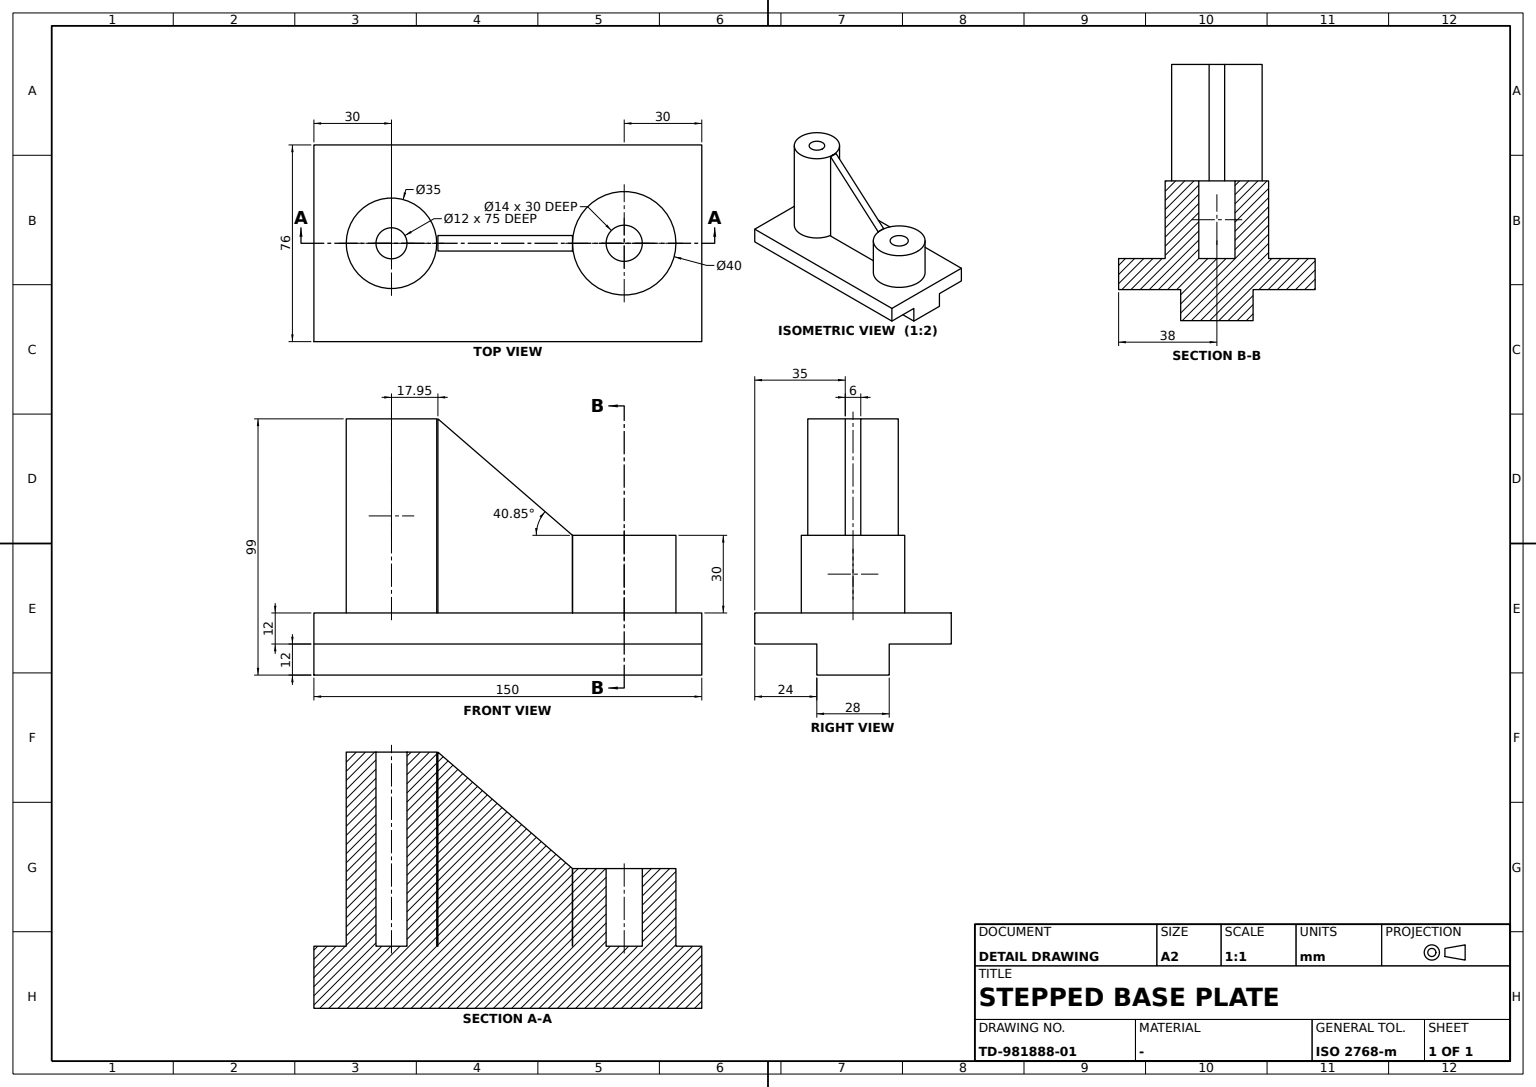
ISO-10303-21;
HEADER;
FILE_DESCRIPTION((''),'2;1');
FILE_NAME('','',(''),(''),'','','');
FILE_SCHEMA(('AUTOMOTIVE_DESIGN'));
ENDSEC;
DATA;
#1=APPLICATION_CONTEXT('');
#2=PRODUCT_CONTEXT('',#1,'mechanical');
#3=PRODUCT('','','',(#2));
#4=PRODUCT_DEFINITION_FORMATION('','',#3);
#5=PRODUCT_DEFINITION_CONTEXT('',#1,'design');
#6=PRODUCT_DEFINITION('','',#4,#5);
#7=PRODUCT_DEFINITION_SHAPE('','',#6);
#8=(LENGTH_UNIT()NAMED_UNIT(*)SI_UNIT(.MILLI.,.METRE.));
#9=(NAMED_UNIT(*)PLANE_ANGLE_UNIT()SI_UNIT($,.RADIAN.));
#10=(NAMED_UNIT(*)SI_UNIT($,.STERADIAN.)SOLID_ANGLE_UNIT());
#11=UNCERTAINTY_MEASURE_WITH_UNIT(LENGTH_MEASURE(0.005),#8,'distance_accuracy_value','');
#12=(GEOMETRIC_REPRESENTATION_CONTEXT(3)GLOBAL_UNCERTAINTY_ASSIGNED_CONTEXT((#11))GLOBAL_UNIT_ASSIGNED_CONTEXT((#8,#9,#10))REPRESENTATION_CONTEXT('',''));
#13=CARTESIAN_POINT('',(-150.,38.,0.));
#14=VERTEX_POINT('',#13);
#15=CARTESIAN_POINT('',(-150.,38.,-12.));
#16=VERTEX_POINT('',#15);
#17=DIRECTION('',(0.,0.,-1.));
#18=VECTOR('',#17,1000.);
#19=LINE('',#13,#18);
#20=EDGE_CURVE('',#14,#16,#19,.T.);
#21=ORIENTED_EDGE('',*,*,#20,.F.);
#22=CARTESIAN_POINT('',(0.,38.,0.));
#23=VERTEX_POINT('',#22);
#24=DIRECTION('',(-1.,0.,0.));
#25=VECTOR('',#24,1000.);
#26=LINE('',#22,#25);
#27=EDGE_CURVE('',#23,#14,#26,.T.);
#28=ORIENTED_EDGE('',*,*,#27,.F.);
#29=CARTESIAN_POINT('',(0.,38.,-12.));
#30=VERTEX_POINT('',#29);
#31=LINE('',#22,#18);
#32=EDGE_CURVE('',#23,#30,#31,.T.);
#33=ORIENTED_EDGE('',*,*,#32,.T.);
#34=LINE('',#29,#25);
#35=EDGE_CURVE('',#30,#16,#34,.T.);
#36=ORIENTED_EDGE('',*,*,#35,.T.);
#37=EDGE_LOOP('',(#21,#28,#33,#36));
#38=FACE_BOUND('',#37,.T.);
#39=DIRECTION('',(0.,1.,0.));
#40=AXIS2_PLACEMENT_3D('',#22,#39,#17);
#41=PLANE('',#40);
#42=ADVANCED_FACE('',(#38),#41,.T.);
#43=CARTESIAN_POINT('',(-102.045097,-3.,0.));
#44=VERTEX_POINT('',#43);
#45=CARTESIAN_POINT('',(-102.045097,3.,0.));
#46=VERTEX_POINT('',#45);
#47=CARTESIAN_POINT('',(-102.045097,0.,0.));
#48=VECTOR('',#39,1000.);
#49=LINE('',#47,#48);
#50=EDGE_CURVE('',#44,#46,#49,.T.);
#51=ORIENTED_EDGE('',*,*,#50,.F.);
#52=CARTESIAN_POINT('',(-102.045097,-3.,75.));
#53=VERTEX_POINT('',#52);
#54=DIRECTION('',(0.,0.,1.));
#55=VECTOR('',#54,1000.);
#56=LINE('',#43,#55);
#57=EDGE_CURVE('',#44,#53,#56,.T.);
#58=ORIENTED_EDGE('',*,*,#57,.T.);
#59=CARTESIAN_POINT('',(-102.045097,3.,75.));
#60=VERTEX_POINT('',#59);
#61=CARTESIAN_POINT('',(-102.045097,0.,75.));
#62=LINE('',#61,#48);
#63=EDGE_CURVE('',#53,#60,#62,.T.);
#64=ORIENTED_EDGE('',*,*,#63,.T.);
#65=LINE('',#45,#55);
#66=EDGE_CURVE('',#46,#60,#65,.T.);
#67=ORIENTED_EDGE('',*,*,#66,.F.);
#68=EDGE_LOOP('',(#51,#58,#64,#67));
#69=FACE_BOUND('',#68,.T.);
#70=AXIS2_PLACEMENT_3D('',#47,#24,#54);
#71=PLANE('',#70);
#72=ADVANCED_FACE('',(#69),#71,.T.);
#73=CARTESIAN_POINT('',(-150.,-38.,0.));
#74=VERTEX_POINT('',#73);
#75=LINE('',#73,#48);
#76=EDGE_CURVE('',#74,#14,#75,.T.);
#77=ORIENTED_EDGE('',*,*,#76,.F.);
#78=CARTESIAN_POINT('',(0.,-38.,0.));
#79=VERTEX_POINT('',#78);
#80=LINE('',#78,#25);
#81=EDGE_CURVE('',#79,#74,#80,.T.);
#82=ORIENTED_EDGE('',*,*,#81,.F.);
#83=LINE('',#78,#48);
#84=EDGE_CURVE('',#79,#23,#83,.T.);
#85=ORIENTED_EDGE('',*,*,#84,.T.);
#86=ORIENTED_EDGE('',*,*,#27,.T.);
#87=EDGE_LOOP('',(#77,#82,#85,#86));
#88=FACE_BOUND('',#87,.T.);
#89=CARTESIAN_POINT('',(-102.5,0.,0.));
#90=VERTEX_POINT('',#89);
#91=CARTESIAN_POINT('',(-120.,0.,0.));
#92=DIRECTION('',(1.,0.,0.));
#93=AXIS2_PLACEMENT_3D('',#91,#54,#92);
#94=CIRCLE('',#93,17.5);
#95=EDGE_CURVE('',#90,#90,#94,.T.);
#96=ORIENTED_EDGE('',*,*,#95,.F.);
#97=EDGE_LOOP('',(#96));
#98=FACE_BOUND('',#97,.T.);
#99=CARTESIAN_POINT('',(-10.,0.,0.));
#100=VERTEX_POINT('',#99);
#101=CARTESIAN_POINT('',(-30.,0.,0.));
#102=AXIS2_PLACEMENT_3D('',#101,#54,#92);
#103=CIRCLE('',#102,20.);
#104=EDGE_CURVE('',#100,#100,#103,.T.);
#105=ORIENTED_EDGE('',*,*,#104,.F.);
#106=EDGE_LOOP('',(#105));
#107=FACE_BOUND('',#106,.T.);
#108=CARTESIAN_POINT('',(-50.001579,-3.,0.));
#109=VERTEX_POINT('',#108);
#110=CARTESIAN_POINT('',(-50.001579,3.,0.));
#111=VERTEX_POINT('',#110);
#112=CARTESIAN_POINT('',(-50.001579,-38.,0.));
#113=LINE('',#112,#48);
#114=EDGE_CURVE('',#109,#111,#113,.T.);
#115=ORIENTED_EDGE('',*,*,#114,.F.);
#116=CARTESIAN_POINT('',(0.,-3.,0.));
#117=LINE('',#116,#25);
#118=EDGE_CURVE('',#109,#44,#117,.T.);
#119=ORIENTED_EDGE('',*,*,#118,.T.);
#120=ORIENTED_EDGE('',*,*,#50,.T.);
#121=CARTESIAN_POINT('',(0.,3.,0.));
#122=LINE('',#121,#25);
#123=EDGE_CURVE('',#111,#46,#122,.T.);
#124=ORIENTED_EDGE('',*,*,#123,.F.);
#125=EDGE_LOOP('',(#115,#119,#120,#124));
#126=FACE_BOUND('',#125,.T.);
#127=AXIS2_PLACEMENT_3D('',#78,#54,#39);
#128=PLANE('',#127);
#129=ADVANCED_FACE('',(#88,#98,#107,#126),#128,.T.);
#130=ORIENTED_EDGE('',*,*,#104,.T.);
#131=EDGE_LOOP('',(#130));
#132=FACE_BOUND('',#131,.T.);
#133=CARTESIAN_POINT('',(-10.,0.,30.));
#134=VERTEX_POINT('',#133);
#135=CARTESIAN_POINT('',(-30.,0.,30.));
#136=AXIS2_PLACEMENT_3D('',#135,#54,#92);
#137=CIRCLE('',#136,20.);
#138=EDGE_CURVE('',#134,#134,#137,.T.);
#139=ORIENTED_EDGE('',*,*,#138,.F.);
#140=EDGE_LOOP('',(#139));
#141=FACE_BOUND('',#140,.T.);
#142=CARTESIAN_POINT('',(-30.,0.,15.));
#143=AXIS2_PLACEMENT_3D('',#142,#54,#92);
#144=CYLINDRICAL_SURFACE('',#143,20.);
#145=ADVANCED_FACE('',(#132,#141),#144,.T.);
#146=ORIENTED_EDGE('',*,*,#114,.T.);
#147=CARTESIAN_POINT('',(-50.001579,3.,30.));
#148=VERTEX_POINT('',#147);
#149=LINE('',#110,#18);
#150=EDGE_CURVE('',#148,#111,#149,.T.);
#151=ORIENTED_EDGE('',*,*,#150,.F.);
#152=CARTESIAN_POINT('',(-50.001579,-3.,30.));
#153=VERTEX_POINT('',#152);
#154=CARTESIAN_POINT('',(-50.001579,0.,30.));
#155=LINE('',#154,#48);
#156=EDGE_CURVE('',#153,#148,#155,.T.);
#157=ORIENTED_EDGE('',*,*,#156,.F.);
#158=LINE('',#108,#18);
#159=EDGE_CURVE('',#153,#109,#158,.T.);
#160=ORIENTED_EDGE('',*,*,#159,.T.);
#161=EDGE_LOOP('',(#146,#151,#157,#160));
#162=FACE_BOUND('',#161,.T.);
#163=AXIS2_PLACEMENT_3D('',#154,#92,#17);
#164=PLANE('',#163);
#165=ADVANCED_FACE('',(#162),#164,.T.);
#166=ORIENTED_EDGE('',*,*,#156,.T.);
#167=CARTESIAN_POINT('',(-6.547854,3.,-7.572741));
#168=DIRECTION('',(0.75643947,0.,-0.654063703));
#169=VECTOR('',#168,1000.);
#170=LINE('',#167,#169);
#171=EDGE_CURVE('',#60,#148,#170,.T.);
#172=ORIENTED_EDGE('',*,*,#171,.F.);
#173=ORIENTED_EDGE('',*,*,#63,.F.);
#174=CARTESIAN_POINT('',(-6.547854,-3.,-7.572741));
#175=LINE('',#174,#169);
#176=EDGE_CURVE('',#53,#153,#175,.T.);
#177=ORIENTED_EDGE('',*,*,#176,.T.);
#178=EDGE_LOOP('',(#166,#172,#173,#177));
#179=FACE_BOUND('',#178,.T.);
#180=DIRECTION('',(0.654063703,0.,0.75643947));
#181=AXIS2_PLACEMENT_3D('',#61,#180,#168);
#182=PLANE('',#181);
#183=ADVANCED_FACE('',(#179),#182,.T.);
#184=CARTESIAN_POINT('',(0.,14.,-12.));
#185=VERTEX_POINT('',#184);
#186=CARTESIAN_POINT('',(-150.,14.,-12.));
#187=VERTEX_POINT('',#186);
#188=LINE('',#184,#25);
#189=EDGE_CURVE('',#185,#187,#188,.T.);
#190=ORIENTED_EDGE('',*,*,#189,.F.);
#191=CARTESIAN_POINT('',(0.,14.,-24.));
#192=VERTEX_POINT('',#191);
#193=LINE('',#184,#18);
#194=EDGE_CURVE('',#185,#192,#193,.T.);
#195=ORIENTED_EDGE('',*,*,#194,.T.);
#196=CARTESIAN_POINT('',(-150.,14.,-24.));
#197=VERTEX_POINT('',#196);
#198=LINE('',#191,#25);
#199=EDGE_CURVE('',#192,#197,#198,.T.);
#200=ORIENTED_EDGE('',*,*,#199,.T.);
#201=LINE('',#186,#18);
#202=EDGE_CURVE('',#187,#197,#201,.T.);
#203=ORIENTED_EDGE('',*,*,#202,.F.);
#204=EDGE_LOOP('',(#190,#195,#200,#203));
#205=FACE_BOUND('',#204,.T.);
#206=AXIS2_PLACEMENT_3D('',#184,#39,#17);
#207=PLANE('',#206);
#208=ADVANCED_FACE('',(#205),#207,.T.);
#209=CARTESIAN_POINT('',(-150.,-14.,-12.));
#210=VERTEX_POINT('',#209);
#211=CARTESIAN_POINT('',(-150.,-38.,-12.));
#212=VERTEX_POINT('',#211);
#213=DIRECTION('',(0.,-1.,0.));
#214=VECTOR('',#213,1000.);
#215=LINE('',#209,#214);
#216=EDGE_CURVE('',#210,#212,#215,.T.);
#217=ORIENTED_EDGE('',*,*,#216,.T.);
#218=LINE('',#211,#55);
#219=EDGE_CURVE('',#212,#74,#218,.T.);
#220=ORIENTED_EDGE('',*,*,#219,.T.);
#221=ORIENTED_EDGE('',*,*,#76,.T.);
#222=ORIENTED_EDGE('',*,*,#20,.T.);
#223=EDGE_CURVE('',#16,#187,#215,.T.);
#224=ORIENTED_EDGE('',*,*,#223,.T.);
#225=ORIENTED_EDGE('',*,*,#202,.T.);
#226=CARTESIAN_POINT('',(-150.,-14.,-24.));
#227=VERTEX_POINT('',#226);
#228=LINE('',#196,#214);
#229=EDGE_CURVE('',#197,#227,#228,.T.);
#230=ORIENTED_EDGE('',*,*,#229,.T.);
#231=LINE('',#226,#55);
#232=EDGE_CURVE('',#227,#210,#231,.T.);
#233=ORIENTED_EDGE('',*,*,#232,.T.);
#234=EDGE_LOOP('',(#217,#220,#221,#222,#224,#225,#230,#233));
#235=FACE_BOUND('',#234,.T.);
#236=CARTESIAN_POINT('',(-150.,0.,0.));
#237=AXIS2_PLACEMENT_3D('',#236,#92,#39);
#238=PLANE('',#237);
#239=ADVANCED_FACE('',(#235),#238,.F.);
#240=ORIENTED_EDGE('',*,*,#223,.F.);
#241=ORIENTED_EDGE('',*,*,#35,.F.);
#242=CARTESIAN_POINT('',(0.,-14.,-12.));
#243=LINE('',#242,#214);
#244=EDGE_CURVE('',#30,#185,#243,.T.);
#245=ORIENTED_EDGE('',*,*,#244,.T.);
#246=ORIENTED_EDGE('',*,*,#189,.T.);
#247=EDGE_LOOP('',(#240,#241,#245,#246));
#248=FACE_BOUND('',#247,.T.);
#249=AXIS2_PLACEMENT_3D('',#242,#17,#213);
#250=PLANE('',#249);
#251=ADVANCED_FACE('',(#248),#250,.T.);
#252=VERTEX_POINT('',#242);
#253=LINE('',#242,#25);
#254=EDGE_CURVE('',#252,#210,#253,.T.);
#255=ORIENTED_EDGE('',*,*,#254,.F.);
#256=CARTESIAN_POINT('',(0.,-38.,-12.));
#257=VERTEX_POINT('',#256);
#258=EDGE_CURVE('',#252,#257,#243,.T.);
#259=ORIENTED_EDGE('',*,*,#258,.T.);
#260=LINE('',#256,#25);
#261=EDGE_CURVE('',#257,#212,#260,.T.);
#262=ORIENTED_EDGE('',*,*,#261,.T.);
#263=ORIENTED_EDGE('',*,*,#216,.F.);
#264=EDGE_LOOP('',(#255,#259,#262,#263));
#265=FACE_BOUND('',#264,.T.);
#266=ADVANCED_FACE('',(#265),#250,.T.);
#267=CARTESIAN_POINT('',(-114.,0.,0.));
#268=VERTEX_POINT('',#267);
#269=CIRCLE('',#93,6.);
#270=EDGE_CURVE('',#268,#268,#269,.T.);
#271=ORIENTED_EDGE('',*,*,#270,.T.);
#272=EDGE_LOOP('',(#271));
#273=FACE_BOUND('',#272,.T.);
#274=ADVANCED_FACE('',(#273),#128,.T.);
#275=CARTESIAN_POINT('',(-23.,0.,30.));
#276=VERTEX_POINT('',#275);
#277=CIRCLE('',#136,7.);
#278=EDGE_CURVE('',#276,#276,#277,.T.);
#279=ORIENTED_EDGE('',*,*,#278,.F.);
#280=EDGE_LOOP('',(#279));
#281=FACE_BOUND('',#280,.T.);
#282=ORIENTED_EDGE('',*,*,#138,.T.);
#283=EDGE_LOOP('',(#282));
#284=FACE_BOUND('',#283,.T.);
#285=CARTESIAN_POINT('',(0.,0.,30.));
#286=AXIS2_PLACEMENT_3D('',#285,#54,#92);
#287=PLANE('',#286);
#288=ADVANCED_FACE('',(#281,#284),#287,.T.);
#289=CARTESIAN_POINT('',(-102.5,0.,75.));
#290=VERTEX_POINT('',#289);
#291=CARTESIAN_POINT('',(-120.,0.,75.));
#292=AXIS2_PLACEMENT_3D('',#291,#54,#92);
#293=CIRCLE('',#292,17.5);
#294=EDGE_CURVE('',#290,#290,#293,.T.);
#295=ORIENTED_EDGE('',*,*,#294,.T.);
#296=EDGE_LOOP('',(#295));
#297=FACE_BOUND('',#296,.T.);
#298=CARTESIAN_POINT('',(-114.,0.,75.));
#299=VERTEX_POINT('',#298);
#300=CIRCLE('',#292,6.);
#301=EDGE_CURVE('',#299,#299,#300,.T.);
#302=ORIENTED_EDGE('',*,*,#301,.F.);
#303=EDGE_LOOP('',(#302));
#304=FACE_BOUND('',#303,.T.);
#305=CARTESIAN_POINT('',(0.,0.,75.));
#306=AXIS2_PLACEMENT_3D('',#305,#54,#92);
#307=PLANE('',#306);
#308=ADVANCED_FACE('',(#297,#304),#307,.T.);
#309=ORIENTED_EDGE('',*,*,#194,.F.);
#310=ORIENTED_EDGE('',*,*,#244,.F.);
#311=ORIENTED_EDGE('',*,*,#32,.F.);
#312=ORIENTED_EDGE('',*,*,#84,.F.);
#313=LINE('',#256,#55);
#314=EDGE_CURVE('',#257,#79,#313,.T.);
#315=ORIENTED_EDGE('',*,*,#314,.F.);
#316=ORIENTED_EDGE('',*,*,#258,.F.);
#317=CARTESIAN_POINT('',(0.,-14.,-24.));
#318=VERTEX_POINT('',#317);
#319=LINE('',#317,#55);
#320=EDGE_CURVE('',#318,#252,#319,.T.);
#321=ORIENTED_EDGE('',*,*,#320,.F.);
#322=LINE('',#191,#214);
#323=EDGE_CURVE('',#192,#318,#322,.T.);
#324=ORIENTED_EDGE('',*,*,#323,.F.);
#325=EDGE_LOOP('',(#309,#310,#311,#312,#315,#316,#321,#324));
#326=FACE_BOUND('',#325,.T.);
#327=CARTESIAN_POINT('',(0.,0.,0.));
#328=AXIS2_PLACEMENT_3D('',#327,#92,#39);
#329=PLANE('',#328);
#330=ADVANCED_FACE('',(#326),#329,.T.);
#331=ORIENTED_EDGE('',*,*,#232,.F.);
#332=LINE('',#317,#25);
#333=EDGE_CURVE('',#318,#227,#332,.T.);
#334=ORIENTED_EDGE('',*,*,#333,.F.);
#335=ORIENTED_EDGE('',*,*,#320,.T.);
#336=ORIENTED_EDGE('',*,*,#254,.T.);
#337=EDGE_LOOP('',(#331,#334,#335,#336));
#338=FACE_BOUND('',#337,.T.);
#339=AXIS2_PLACEMENT_3D('',#317,#213,#54);
#340=PLANE('',#339);
#341=ADVANCED_FACE('',(#338),#340,.T.);
#342=ORIENTED_EDGE('',*,*,#270,.F.);
#343=EDGE_LOOP('',(#342));
#344=FACE_BOUND('',#343,.T.);
#345=ORIENTED_EDGE('',*,*,#301,.T.);
#346=EDGE_LOOP('',(#345));
#347=FACE_BOUND('',#346,.T.);
#348=CARTESIAN_POINT('',(-120.,0.,24.84));
#349=AXIS2_PLACEMENT_3D('',#348,#54,#92);
#350=CYLINDRICAL_SURFACE('',#349,6.);
#351=ADVANCED_FACE('',(#344,#347),#350,.F.);
#352=CARTESIAN_POINT('',(-23.,0.,0.));
#353=VERTEX_POINT('',#352);
#354=CIRCLE('',#102,7.);
#355=EDGE_CURVE('',#353,#353,#354,.T.);
#356=ORIENTED_EDGE('',*,*,#355,.T.);
#357=EDGE_LOOP('',(#356));
#358=FACE_BOUND('',#357,.T.);
#359=ADVANCED_FACE('',(#358),#128,.T.);
#360=ORIENTED_EDGE('',*,*,#261,.F.);
#361=ORIENTED_EDGE('',*,*,#314,.T.);
#362=ORIENTED_EDGE('',*,*,#81,.T.);
#363=ORIENTED_EDGE('',*,*,#219,.F.);
#364=EDGE_LOOP('',(#360,#361,#362,#363));
#365=FACE_BOUND('',#364,.T.);
#366=AXIS2_PLACEMENT_3D('',#256,#213,#54);
#367=PLANE('',#366);
#368=ADVANCED_FACE('',(#365),#367,.T.);
#369=ORIENTED_EDGE('',*,*,#95,.T.);
#370=EDGE_LOOP('',(#369));
#371=FACE_BOUND('',#370,.T.);
#372=ORIENTED_EDGE('',*,*,#294,.F.);
#373=EDGE_LOOP('',(#372));
#374=FACE_BOUND('',#373,.T.);
#375=CYLINDRICAL_SURFACE('',#349,17.5);
#376=ADVANCED_FACE('',(#371,#374),#375,.T.);
#377=ORIENTED_EDGE('',*,*,#355,.F.);
#378=EDGE_LOOP('',(#377));
#379=FACE_BOUND('',#378,.T.);
#380=ORIENTED_EDGE('',*,*,#278,.T.);
#381=EDGE_LOOP('',(#380));
#382=FACE_BOUND('',#381,.T.);
#383=CYLINDRICAL_SURFACE('',#143,7.);
#384=ADVANCED_FACE('',(#379,#382),#383,.F.);
#385=ORIENTED_EDGE('',*,*,#66,.T.);
#386=ORIENTED_EDGE('',*,*,#171,.T.);
#387=ORIENTED_EDGE('',*,*,#150,.T.);
#388=ORIENTED_EDGE('',*,*,#123,.T.);
#389=EDGE_LOOP('',(#385,#386,#387,#388));
#390=FACE_BOUND('',#389,.T.);
#391=AXIS2_PLACEMENT_3D('',#121,#39,#24);
#392=PLANE('',#391);
#393=ADVANCED_FACE('',(#390),#392,.T.);
#394=ORIENTED_EDGE('',*,*,#333,.T.);
#395=ORIENTED_EDGE('',*,*,#229,.F.);
#396=ORIENTED_EDGE('',*,*,#199,.F.);
#397=ORIENTED_EDGE('',*,*,#323,.T.);
#398=EDGE_LOOP('',(#394,#395,#396,#397));
#399=FACE_BOUND('',#398,.T.);
#400=AXIS2_PLACEMENT_3D('',#191,#17,#213);
#401=PLANE('',#400);
#402=ADVANCED_FACE('',(#399),#401,.T.);
#403=ORIENTED_EDGE('',*,*,#118,.F.);
#404=ORIENTED_EDGE('',*,*,#159,.F.);
#405=ORIENTED_EDGE('',*,*,#176,.F.);
#406=ORIENTED_EDGE('',*,*,#57,.F.);
#407=EDGE_LOOP('',(#403,#404,#405,#406));
#408=FACE_BOUND('',#407,.T.);
#409=AXIS2_PLACEMENT_3D('',#116,#39,#24);
#410=PLANE('',#409);
#411=ADVANCED_FACE('',(#408),#410,.F.);
#412=CLOSED_SHELL('',(#42,#72,#129,#145,#165,#183,#208,#239,#251,#266,#274,#288,#308,#330,#341,#351,#359,#368,#376,#384,#393,#402,#411));
#413=MANIFOLD_SOLID_BREP('',#412);
#414=ADVANCED_BREP_SHAPE_REPRESENTATION('',(#413),#12);
#415=SHAPE_DEFINITION_REPRESENTATION(#7,#414);
ENDSEC;
END-ISO-10303-21;
